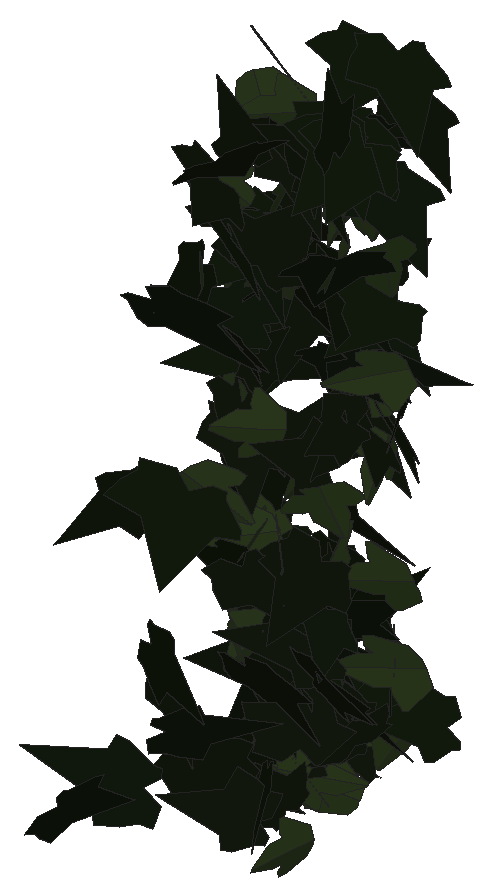
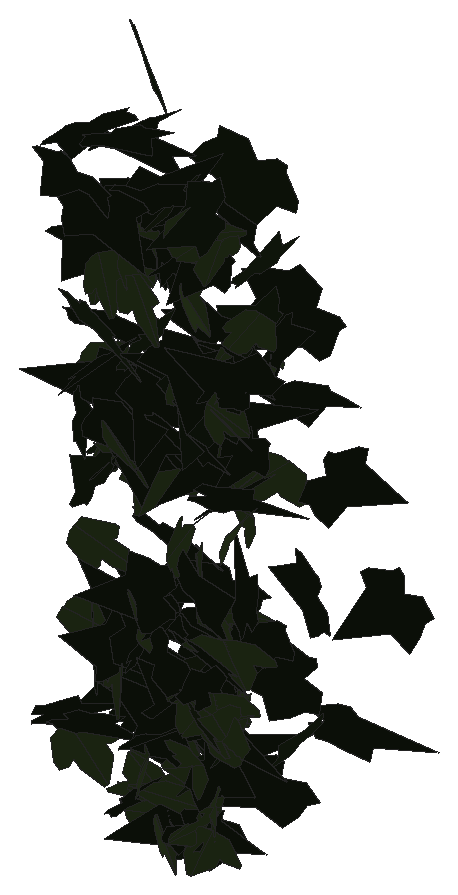
# SketchUp Ruby script. Lengths in inches.
U = 1.inch
M = Sketchup.active_model
def pt(a) = Geom::Point3d.new(a.map { |v| v * U })
def face(e, loops, mat)
  f = e.add_face(loops[0].map { |a| pt(a) })
  loops[1..].each { |l| e.add_face(l.map { |a| pt(a) }).erase! }
  f.material = f.back_material = mat if mat
  f
end
# faces: each face lists its corners as indices into pts; further lists are holes
def faces(e, pts, list, mat = nil) = list.each { |f| face(e, (f[0].is_a?(Array) ? f : [f]).map { |l| l.map { |i| pts[i] } }, mat) }
# xy, xz, yz: faces in a plane at the given z, y or x. An outline is a flat list of corners, or four numbers for a rectangle; further outlines are holes
def ring(l) = l.size == 4 ? [[l[0], l[1]], [l[2], l[1]], [l[2], l[3]], [l[0], l[3]]] : l.each_slice(2).to_a
def flat(e, list, mat, &to3) = list.each { |f| face(e, (f[0].is_a?(Array) ? f : [f]).map { |l| ring(l).map { |u, v| to3.(u, v) } }, mat) }
def xy(e, z, list, mat = nil) = flat(e, list, mat) { |x, y| [x, y, z] }
def xz(e, y, list, mat = nil) = flat(e, list, mat) { |x, z| [x, y, z] }
def yz(e, x, list, mat = nil) = flat(e, list, mat) { |y, z| [x, y, z] }
def lines(e, pts, list) = list.each { |a, b| e.add_line(pt(pts[a]), pt(pts[b])) }
# prism: a flat outline (further loops are holes) pulled along v
def prism(e, loops, v, mat = nil)
  f = face(e, loops, mat); d = Geom::Vector3d.new(v.map { |x| x * U })
  f.pushpull(f.normal.samedirection?(d) ? d.length : -d.length)
end
def box(e, o, s, mat = nil) = prism(e, [[o, [o[0] + s[0], o[1], o[2]], [o[0] + s[0], o[1] + s[1], o[2]], [o[0], o[1] + s[1], o[2]]]], [0, 0, s[2]], mat)
def at(x, y, z, deg = 0) = Geom::Transformation.translation(pt([x, y, z])) * Geom::Transformation.rotation(ORIGIN, Z_AXIS, deg.degrees)
def axes(o, x, y, z) = Geom::Transformation.new([*x, 0, *y, 0, *z, 0, *pt(o).to_a, 1])
def part(name) = M.definitions.add(name)
# library, detail: a bought-in or finely detailed component or shape, given as its bounding box
def library(name, o, s) = part(name).tap { |d| box(d.entities, o, s) }
def detail(e, o, s) = box(e.add_group.entities, o, s)
def put(e, d, t, mat = nil) = e.add_instance(d, t).tap { |i| i.material = mat if mat }
def group(e, t, mat = nil) = e.add_group.tap { |g| g.transformation = t; g.material = mat if mat }.entities
root = M.entities
M.materials.add("1026 AP 7946 SUNNY SIDE UP").color = [254, 231, 186]
M.materials.add("efeu1").color = [18, 25, 13]
M.materials.add("efeu2").color = [43, 57, 29]
c1 = part("ivyleaf_9")
p = [[1.54,2.16,1.25],[1.36,2.04,1.19],[-0.21,0.99,0.68],[-0.71,1.11,0.82],[-0.85,0.86,0.67],[-0.8,0.17,0.21],
  [-0.9,-0.01,0.1],[-0.67,-0.16,-0.02],[-0.08,-0.08,-0.05],[-0.03,-0.6,-0.4],[0.65,-0.88,-0.66],[0.83,-0.6,-0.49],
  [1.29,-0.42,-0.43],[1.8125,-0.07,-0.26],[1.21,0.44,0.15]]
faces(c1.entities,p,[[0,1,2,3,4,5,6,7,8,9,10,11,12,13,14]],"efeu1")
c2 = part("ivyleaf_10")
p = [[0,0.5,-0.03],[-0.0625,2.02,-0.43],[-0.19,2.01,-0.46],[-0.54,1.05,-0.29],[-0.52,0.625,-0.18],[-0.83,0.76,-0.28],
  [-1.16,0.64,-0.33],[-1.15,0.33,-0.24],[-0.77,-0.39,0.02],[-0.3,-0.51,0.16],[0.04,-0.48,0.23],[-0.02,2.01,-0.4375],
  [-0.06,2.01,-0.43],[0.04,-0.49,0.23],[0.67,-0.49,0.14],[1.38,0.36,-0.2],[1.375,0.51,-0.24],[0.81,0.65,-0.19],
  [0.62,0.59,-0.15],[0.6,1.09,-0.28],[0.5,1.23,-0.31]]
faces(c2.entities,p,[[0,1,2,3,4,5,6,7,8,9,10],[11,12,0,13,14,15,16,17,18,19,20]],"efeu2")
put(root,c1,axes([137.74,211.1,285.49],[-0.46349,-0.03246,0.23441],[-0.33897,-0.09016,-0.30122],[0.12619,-0.36141,0.05183]),"1026 AP 7946 SUNNY SIDE UP")
put(root,c2,axes([137.5625,210.79,284.78],[-0.00796,0.33057,-0.23303],[-0.14205,0.22131,0.33381],[0.61532,0.05537,0.07405]),"1026 AP 7946 SUNNY SIDE UP")
put(root,c1,axes([137.1875,210.96,283.58],[-0.03472,0.01197,0.4574],[0.05164,-0.44321,0.0114],[0.69637,0.03346,0.02196]),"1026 AP 7946 SUNNY SIDE UP")
put(root,c2,axes([137.37,211.12,283.06],[0.60482,0.09796,-0.04757],[-0.05306,-0.05562,-0.40657],[-0.1622,0.38346,-0.04438]),"1026 AP 7946 SUNNY SIDE UP")
put(root,c1,axes([137.98,208,280.22],[-0.34427,-0.14792,-0.33556],[-0.41907,-0.18582,0.2711],[-0.37342,0.3449,0.00512]),"1026 AP 7946 SUNNY SIDE UP")
put(root,c2,axes([137.5,211.23,287.08],[-0.01346,-0.25376,0.25977],[0.0236,-0.25371,-0.26249],[0.56362,0.00456,0.01719]),"1026 AP 7946 SUNNY SIDE UP")
put(root,c2,axes([137.33,210.61,288.33],[-0.17262,-0.24856,-0.23455],[0.26251,0.16626,-0.27064],[0.45871,-0.18869,0.06662]),"1026 AP 7946 SUNNY SIDE UP")
put(root,c1,axes([137.17,210.98,287.41],[-0.08394,0.02556,0.38678],[0.58508,0.05924,0.05072],[-0.08684,0.37442,-0.03217]),"1026 AP 7946 SUNNY SIDE UP")
put(root,c1,axes([137.31,209.54,280.79],[0.11048,-0.33291,0.09369],[0.01592,-0.09271,-0.35094],[0.54321,0.07043,-0.00877]),"1026 AP 7946 SUNNY SIDE UP")
put(root,c1,axes([137.71,208.33,284.62],[-0.11173,0.01078,-0.43675],[0.14962,-0.41855,-0.02984],[-0.64992,-0.09821,0.06821]),"1026 AP 7946 SUNNY SIDE UP")
put(root,c2,axes([137.57,211.21,281.84],[0.26628,0.25014,-0.15649],[-0.10126,-0.14103,-0.31112],[-0.45008,0.17972,-0.02259]),"1026 AP 7946 SUNNY SIDE UP")
put(root,c1,axes([138,210.9375,286.89],[-0.51521,0.09643,-0.21913],[-0.30085,0.10094,0.35046],[0.21195,0.37768,-0.03521]),"1026 AP 7946 SUNNY SIDE UP")
put(root,c2,axes([137.84,210.37,281.32],[-0.26236,0.30006,-0.21856],[-0.13006,0.19827,0.35423],[0.5646,0.1851,-0.01996]),"1026 AP 7946 SUNNY SIDE UP")
put(root,c1,axes([137.79,211.36,282.19],[0.00629,0.06183,0.33107],[-0.3689,-0.22304,0.04596],[0.35799,-0.23092,0.04155]),"1026 AP 7946 SUNNY SIDE UP")
put(root,c1,axes([138.09,210.49,286.42],[-0.18557,0.01426,0.38117],[-0.57425,-0.068,-0.11773],[0.09522,-0.38228,0.03285]),"1026 AP 7946 SUNNY SIDE UP")
put(root,c1,axes([137.62,210.12,282.93],[0.4821,0.12099,-0.13652],[-0.17707,-0.07626,-0.33883],[-0.2207,0.32547,-0.02637]),"1026 AP 7946 SUNNY SIDE UP")
put(root,c2,axes([137.47,210.6,285.07],[-0.18929,0.09258,-0.32433],[0.22353,-0.28813,-0.14474],[-0.46595,-0.17584,0.06232]),"1026 AP 7946 SUNNY SIDE UP")
put(root,c2,axes([137.86,211.07,281.86],[-0.39768,-0.24134,0.12812],[-0.11078,-0.10773,-0.35965],[0.41332,-0.26109,0.02688]),"1026 AP 7946 SUNNY SIDE UP")
put(root,c1,axes([137.63,209.79,287.46],[0.00424,-0.13917,-0.37407],[0.33016,-0.3042,0.1202],[-0.51327,-0.19682,0.07423]),"1026 AP 7946 SUNNY SIDE UP")
put(root,c2,axes([137.91,210.87,280],[-0.05666,0.08282,-0.37031],[-0.16778,0.34388,0.09453],[0.55598,0.11222,-0.00921]),"1026 AP 7946 SUNNY SIDE UP")
put(root,c1,axes([137.61,210.34,286.16],[0.50574,-0.0435,-0.13904],[-0.21337,0.00059,-0.33394],[0.06345,0.34871,-0.01471]),"1026 AP 7946 SUNNY SIDE UP")
put(root,c2,axes([137.64,211.06,289.73],[0.18859,0.35281,0.01986],[0.01968,0.01398,-0.38373],[-0.55507,0.12037,-0.00686]),"1026 AP 7946 SUNNY SIDE UP")
put(root,c1,axes([138.07,211.02,283.59],[0.04291,-0.00334,0.42526],[-0.24974,0.38178,0.01623],[-0.59916,-0.15937,0.02369]),"1026 AP 7946 SUNNY SIDE UP")
put(root,c2,axes([137.67,211.05,282.04],[0.54775,0.17392,-0.01781],[-0.00199,-0.03822,-0.39984],[-0.27498,0.34673,-0.03258]),"1026 AP 7946 SUNNY SIDE UP")
put(root,c2,axes([137.9,209.42,287.41],[0.04226,-0.17147,-0.32584],[-0.07619,0.31157,-0.17698],[0.55921,0.05541,0.00051]),"1026 AP 7946 SUNNY SIDE UP")
put(root,c2,axes([137.43,210.99,281.28],[-0.20885,0.03231,0.32991],[0.50582,0.01529,0.13602],[-0.00285,0.34619,-0.03476]),"1026 AP 7946 SUNNY SIDE UP")
put(root,c2,axes([137.77,211.15,279.69],[-0.47179,-0.05614,-0.07473],[0.12212,-0.02547,-0.31213],[0.076,-0.30756,0.03762]),"1026 AP 7946 SUNNY SIDE UP")
put(root,c1,axes([138.03,211.19,282.91],[-0.54347,0.02864,-0.07825],[0.11337,-0.04587,-0.35531],[-0.05918,-0.35093,0.03796]),"1026 AP 7946 SUNNY SIDE UP")
put(root,c1,axes([137.87,211.36,281.94],[-0.36309,0.0419,-0.23239],[0.30878,-0.13005,-0.23248],[-0.18728,-0.29564,0.06723]),"1026 AP 7946 SUNNY SIDE UP")
put(root,c2,axes([138.13,210.52,283.14],[-0.19304,0.03837,0.32138],[-0.25404,-0.29475,-0.0299],[0.42353,-0.1593,0.12855]),"1026 AP 7946 SUNNY SIDE UP")
put(root,c1,axes([138.11,210.84,287.74],[-0.6507,-0.11066,0.00159],[0.00984,-0.0318,-0.44023],[0.17376,-0.41261,0.0309]),"1026 AP 7946 SUNNY SIDE UP")
put(root,c1,axes([137.81,209.9375,288.78],[-0.16803,-0.25295,0.30816],[-0.00825,-0.31054,-0.27298],[0.61765,-0.07296,0.08019]),"1026 AP 7946 SUNNY SIDE UP")
put(root,c1,axes([137.56,210.3,287.93],[0.16366,-0.34602,0.26263],[0.15136,-0.23894,-0.37312],[0.66051,0.14049,0.02043]),"1026 AP 7946 SUNNY SIDE UP")
put(root,c2,axes([138.01,210.58,283.14],[0.15388,-0.36609,-0.06355],[-0.04168,0.05459,-0.38989],[0.58173,0.10075,-0.01113]),"1026 AP 7946 SUNNY SIDE UP")
put(root,c1,axes([137.94,210.94,280.86],[-0.13543,0.10288,-0.42709],[0.34317,-0.35365,-0.139],[-0.57841,-0.23391,0.01753]),"1026 AP 7946 SUNNY SIDE UP")
put(root,c1,axes([138.2,211.0625,279.73],[-0.10653,-0.00302,-0.32575],[-0.11717,-0.31411,0.01771],[-0.4832,0.07683,0.06753]),"1026 AP 7946 SUNNY SIDE UP")
put(root,c1,axes([137.95,211.05,287.76],[0.42562,0.25309,-0.12633],[-0.11842,-0.10082,-0.38173],[-0.42709,0.28017,-0.02006]),"1026 AP 7946 SUNNY SIDE UP")
put(root,c2,axes([137.85,210.93,279.84],[0.01901,-0.06443,-0.35492],[0.23727,0.31169,-0.05283],[0.49679,-0.1464,0.03882]),"1026 AP 7946 SUNNY SIDE UP")
put(root,c1,axes([137.66,211.17,290.33],[0.54574,-0.24878,-0.01932],[-0.05294,-0.0173,-0.43865],[0.38854,0.34708,-0.03263]),"1026 AP 7946 SUNNY SIDE UP")
put(root,c1,axes([138.48,210.42,281.23],[-0.08506,-0.04199,-0.40993],[-0.57758,-0.15339,0.06727],[-0.24852,0.37087,-0.01602]),"1026 AP 7946 SUNNY SIDE UP")
put(root,c2,axes([138.0625,210.62,281.58],[-0.09645,-0.19244,0.31027],[0.01895,-0.3076,-0.20103],[0.56313,-0.02261,0.0599]),"1026 AP 7946 SUNNY SIDE UP")
put(root,c1,axes([138.08,210.75,286.9],[0.14822,0.3837,0.18189],[0.08509,0.16619,-0.40588],[-0.65722,0.10805,-0.01153]),"1026 AP 7946 SUNNY SIDE UP")
put(root,c1,axes([137.78,210.375,285.3],[0.22904,-0.3355,-0.12077],[-0.05452,0.11061,-0.37596],[0.55516,0.14928,0.0129]),"1026 AP 7946 SUNNY SIDE UP")
put(root,c1,axes([138.3125,209.92,289.4],[0.09608,0.05621,0.36297],[-0.23109,0.32935,-0.02597],[-0.51066,-0.13847,0.08004]),"1026 AP 7946 SUNNY SIDE UP")
put(root,c1,axes([138.01,210.67,285.83],[0.07852,-0.02055,-0.36096],[-0.15318,0.33907,-0.03282],[0.53002,0.10104,0.04399]),"1026 AP 7946 SUNNY SIDE UP")
put(root,c1,axes([137.65,210.99,287.45],[0.27573,0.08668,-0.33673],[0.37047,0.23356,0.19509],[0.38246,-0.28872,0.05378]),"1026 AP 7946 SUNNY SIDE UP")
put(root,c1,axes([137.95,210.78,289.38],[0.53423,-0.05838,-0.08906],[-0.14166,-0.01799,-0.35371],[0.08182,0.35003,-0.03092]),"1026 AP 7946 SUNNY SIDE UP")
put(root,c2,axes([137.92,211.3125,280.97],[-0.28853,0.08538,-0.2564],[0.28985,-0.17561,-0.20271],[-0.29625,-0.25498,0.05139]),"1026 AP 7946 SUNNY SIDE UP")
put(root,c2,axes([138.37,210.98,289.62],[0.00829,0.01832,0.40061],[-0.19114,-0.36927,0.01747],[0.58135,-0.12167,0.00003]),"1026 AP 7946 SUNNY SIDE UP")
put(root,c2,axes([138.23,210.9375,287.19],[-0.19891,-0.36412,-0.07047],[0.04199,0.06095,-0.39672],[0.58045,-0.12919,0.00455]),"1026 AP 7946 SUNNY SIDE UP")
put(root,c1,axes([137.81,209.45,279.97],[0.05638,-0.02642,-0.44343],[0.26148,0.3992,-0.00864],[0.62538,-0.16453,0.04359]),"1026 AP 7946 SUNNY SIDE UP")
put(root,c1,axes([137.98,210.57,287.5625],[0.13358,-0.35145,0.02725],[-0.00048,-0.02933,-0.37259],[0.55443,0.08465,-0.00689]),"1026 AP 7946 SUNNY SIDE UP")
put(root,c1,axes([138.23,211.26,286.46],[-0.48512,-0.08538,-0.22038],[0.34945,-0.01945,-0.32305],[0.09241,-0.37465,0.06469]),"1026 AP 7946 SUNNY SIDE UP")
put(root,c1,axes([137.88,208.56,287.51],[0.69955,0.07432,0.10059],[0.162,-0.02968,-0.46251],[-0.10383,0.45442,-0.04392]),"1026 AP 7946 SUNNY SIDE UP")
put(root,c2,axes([138.3,210.92,288.6],[0.15943,-0.31654,0.12841],[0.03367,-0.12575,-0.34272],[0.53492,0.10226,-0.0167]),"1026 AP 7946 SUNNY SIDE UP")
put(root,c1,axes([138.03,210.87,280.66],[0.12269,-0.3446,0.15747],[0.0399,-0.15294,-0.36479],[0.59268,0.08163,-0.00804]),"1026 AP 7946 SUNNY SIDE UP")
put(root,c1,axes([138.14,210.1,284.91],[-0.04201,-0.40238,0.06028],[-0.0018,-0.06085,-0.41579],[0.63989,-0.02659,0.00279]),"1026 AP 7946 SUNNY SIDE UP")
put(root,c1,axes([138.02,211.01,279.68],[0.27349,-0.247,0.17069],[0.12197,-0.14931,-0.31142],[0.45276,0.18942,-0.01921]),"1026 AP 7946 SUNNY SIDE UP")
put(root,c1,axes([138.01,210.78,279.81],[0.04963,0.06052,-0.43509],[0.24736,0.39237,0.07227],[0.62417,-0.16031,0.00596]),"1026 AP 7946 SUNNY SIDE UP")
put(root,c2,axes([138.12,210.86,280],[-0.09705,-0.06156,0.38371],[0.43429,0.25044,0.09118],[-0.40546,0.28298,0.00581]),"1026 AP 7946 SUNNY SIDE UP")
put(root,c1,axes([138.29,210.7,281.47],[-0.26941,-0.02034,0.37963],[0.57082,0.0646,0.17788],[-0.10554,0.40132,-0.00698]),"1026 AP 7946 SUNNY SIDE UP")
put(root,c2,axes([138.31,208.85,284.75],[-0.36463,-0.17551,-0.27318],[0.39901,0.09365,-0.29303],[0.29918,-0.33881,0.05786]),"1026 AP 7946 SUNNY SIDE UP")
put(root,c1,axes([138.34,210.21,287.59],[-0.38467,0.15873,0.32272],[0.41895,-0.16314,0.29942],[0.3578,0.36167,-0.00363]),"1026 AP 7946 SUNNY SIDE UP")
put(root,c2,axes([138.61,211.17,279.61],[0.10706,-0.32773,0.00456],[-0.00681,-0.00732,-0.34483],[0.51538,0.06798,-0.00551]),"1026 AP 7946 SUNNY SIDE UP")
put(root,c1,axes([138.52,205.625,281.125],[-0.09422,0.14745,-0.41655],[-0.16546,0.3917,0.16517],[0.65748,0.1197,-0.01813]),"1026 AP 7946 SUNNY SIDE UP")
put(root,c1,axes([138.13,208.15,282.375],[0.10144,-0.10996,-0.41829],[0.65593,-0.0314,0.07697],[-0.07758,-0.40931,0.10389]),"1026 AP 7946 SUNNY SIDE UP")
put(root,c1,axes([138.65,208.91,289.84],[0.25671,0.43507,0.10699],[0.03686,0.09945,-0.47796],[-0.70146,0.16444,0.01404]),"1026 AP 7946 SUNNY SIDE UP")
put(root,c1,axes([138.26,208.35,281.02],[0.19599,0.25139,-0.30089],[0.11421,0.28765,0.28728],[0.59681,-0.1376,0.04384]),"1026 AP 7946 SUNNY SIDE UP")
put(root,c1,axes([138.47,210.72,289.17],[0.04945,-0.37759,-0.09211],[-0.01641,0.0867,-0.38981],[0.60915,0.03299,-0.00302]),"1026 AP 7946 SUNNY SIDE UP")
put(root,c2,axes([138.54,210.98,279.58],[0.30755,-0.16365,0.19821],[0.22564,-0.1297,-0.26341],[0.3282,0.24252,-0.00465]),"1026 AP 7946 SUNNY SIDE UP")
put(root,c2,axes([138.61,210.85,284.1],[0.00815,0.04029,0.39135],[0.25243,-0.34472,0.03341],[0.54466,0.15916,-0.02134]),"1026 AP 7946 SUNNY SIDE UP")
put(root,c2,axes([138.88,209.71,285.39],[-0.01957,0.11291,0.37513],[-0.09835,-0.35935,0.11068],[0.59037,-0.05612,0.03087]),"1026 AP 7946 SUNNY SIDE UP")
put(root,c1,axes([138.68,211.08,281.1],[-0.20491,-0.35436,-0.05746],[0.05061,0.0454,-0.38842],[0.5613,-0.13346,0.01405]),"1026 AP 7946 SUNNY SIDE UP")
put(root,c1,axes([138.35,211.05,281.26],[0.50353,0.03211,-0.2416],[0.34482,0.10906,0.32425],[0.14086,-0.38176,0.06988]),"1026 AP 7946 SUNNY SIDE UP")
put(root,c2,axes([139.16,211.12,288.5],[-0.40844,0.14317,0.23688],[-0.36623,0.04242,-0.29908],[-0.21529,-0.34376,0.05936]),"1026 AP 7946 SUNNY SIDE UP")
put(root,c1,axes([139.23,208.99,279.7],[-0.18214,-0.01626,0.37054],[-0.51746,-0.14873,-0.11695],[0.23002,-0.34746,0.03031]),"1026 AP 7946 SUNNY SIDE UP")
put(root,c1,axes([138.58,209.6,283.12],[-0.05901,-0.1318,-0.34169],[0.33712,0.25738,-0.12914],[0.44728,-0.21138,0.05226]),"1026 AP 7946 SUNNY SIDE UP")
put(root,c1,axes([138.93,210.82,286.75],[0.53076,-0.034,-0.26208],[-0.39818,0.02242,-0.34936],[0.06393,0.42197,-0.00007]),"1026 AP 7946 SUNNY SIDE UP")
put(root,c1,axes([139.01,211.3,282.42],[-0.11865,-0.05065,0.34679],[-0.24603,-0.30138,-0.08454],[0.47587,-0.16844,0.04276]),"1026 AP 7946 SUNNY SIDE UP")
put(root,c2,axes([138.7,210.11,283.32],[-0.01036,0.05558,0.36623],[0.39402,-0.25401,0.04425],[0.40532,0.24834,-0.03366]),"1026 AP 7946 SUNNY SIDE UP")
put(root,c1,axes([138.73,210.39,281.79],[0.09108,-0.33774,0.17569],[0.05595,-0.16885,-0.35396],[0.59367,0.06773,0.0064]),"1026 AP 7946 SUNNY SIDE UP")
put(root,c2,axes([138.92,211.26,280.67],[-0.2792,0.31833,-0.13124],[0.05096,-0.12927,-0.37475],[-0.53779,-0.17751,0.03262]),"1026 AP 7946 SUNNY SIDE UP")
put(root,c2,axes([139.35,210.73,279.4],[0.09615,0.09084,0.3421],[-0.44286,-0.17986,0.10323],[0.30995,-0.28517,0.04136]),"1026 AP 7946 SUNNY SIDE UP")
put(root,c1,axes([138.55,211.2,282.625],[-0.02312,-0.05097,-0.44311],[0.63311,0.15624,-0.03236],[0.24979,-0.40071,0.04101]),"1026 AP 7946 SUNNY SIDE UP")
put(root,c2,axes([138.84,210.96,280.1],[0.47203,0.16145,-0.18032],[0.20946,0.12136,0.34956],[0.31164,-0.32611,0.03817]),"1026 AP 7946 SUNNY SIDE UP")
put(root,c2,axes([138.96,211.1,282.8],[0.30047,-0.31017,0.07934],[-0.03649,0.07808,0.37516],[-0.50187,-0.19138,0.02023]),"1026 AP 7946 SUNNY SIDE UP")
put(root,c1,axes([138.62,211.22,283.54],[0.49627,-0.12807,0.17797],[0.23457,-0.09238,-0.35038],[0.24482,0.3481,-0.02505]),"1026 AP 7946 SUNNY SIDE UP")
put(root,c1,axes([139.11,207.64,285.35],[-0.51297,-0.30437,-0.11372],[0.18048,0.03521,-0.45642],[0.47505,-0.34204,0.0506]),"1026 AP 7946 SUNNY SIDE UP")
put(root,c1,axes([139.2,211.3,279.91],[-0.2026,-0.21398,0.24257],[-0.17411,-0.20939,-0.25836],[0.47052,-0.16962,0.00884]),"1026 AP 7946 SUNNY SIDE UP")
put(root,c2,axes([138.72,210.53,279.61],[0.08127,-0.06544,-0.35757],[0.5542,-0.00685,0.05542],[-0.02601,-0.35048,0.06356]),"1026 AP 7946 SUNNY SIDE UP")
put(root,c1,axes([138.93,209.24,281.84],[0.67435,-0.01437,-0.05097],[-0.0794,-0.03826,-0.44039],[0.01548,0.43,-0.03835]),"1026 AP 7946 SUNNY SIDE UP")
put(root,c1,axes([139.36,210.87,286.08],[0.4372,0.16547,-0.24735],[-0.29622,-0.15298,-0.33296],[-0.35156,0.33468,-0.02705]),"1026 AP 7946 SUNNY SIDE UP")
put(root,c1,axes([139.79,209.87,282.15],[-0.45597,0.10456,0.26977],[-0.41598,0.02664,-0.31331],[-0.15088,-0.38941,0.04855]),"1026 AP 7946 SUNNY SIDE UP")
put(root,c1,axes([139.51,210.43,289.4375],[0.01085,0.0372,0.45125],[-0.5692,-0.24771,0.02611],[0.39162,-0.36107,0.02545]),"1026 AP 7946 SUNNY SIDE UP")
put(root,c1,axes([139.19,209.28,280.25],[-0.22179,0.0379,-0.33948],[0.45133,-0.16598,-0.14712],[-0.26207,-0.31793,0.03394]),"1026 AP 7946 SUNNY SIDE UP")
put(root,c1,axes([139.61,209.17,279.95],[-0.08431,0.22915,0.28518],[-0.1569,0.25802,-0.23958],[-0.5412,-0.1105,0.02503]),"1026 AP 7946 SUNNY SIDE UP")
put(root,c1,axes([139.22,209.97,284.97],[-0.39456,0.32521,0.16515],[0.18786,-0.10753,0.42162],[0.53692,0.27661,-0.02616]),"1026 AP 7946 SUNNY SIDE UP")
put(root,c2,axes([139.62,210.96,281.93],[-0.28752,0.21273,0.24915],[-0.28296,0.1615,-0.28701],[-0.41832,-0.25546,0.02289]),"1026 AP 7946 SUNNY SIDE UP")
put(root,c2,axes([139.23,211.13,285.44],[0.5052,-0.19909,-0.0787],[0.14235,0.00449,0.38592],[-0.30289,-0.32996,0.0501]),"1026 AP 7946 SUNNY SIDE UP")
put(root,c1,axes([139.65,209.95,284.97],[-0.08654,-0.00456,0.36405],[-0.43184,-0.22458,-0.04836],[0.34981,-0.27837,0.03036]),"1026 AP 7946 SUNNY SIDE UP")
put(root,c1,axes([139.17,210.1875,289.58],[0.24612,-0.37953,0.04675],[0.00843,-0.04918,-0.42298],[0.60137,0.15602,-0.01321]),"1026 AP 7946 SUNNY SIDE UP")
put(root,c1,axes([139.31,210.76,287.29],[-0.02712,-0.30895,0.31104],[0.0054,-0.304,-0.3202],[0.68115,-0.00989,0.01492]),"1026 AP 7946 SUNNY SIDE UP")
put(root,c2,axes([139.5,210.79,288.84],[0.00012,-0.31615,0.23223],[0.0927,-0.22459,-0.32326],[0.60513,0.03447,0.04947]),"1026 AP 7946 SUNNY SIDE UP")
put(root,c1,axes([139.37,210.72,289.9],[-0.19872,-0.36804,-0.17816],[0.09616,0.15962,-0.39991],[0.63074,-0.14029,0.00484]),"1026 AP 7946 SUNNY SIDE UP")
put(root,c1,axes([139.6,209.5,280.79],[-0.42567,-0.14129,0.32846],[0.43176,0.16411,0.31528],[-0.33992,0.38539,-0.01086]),"1026 AP 7946 SUNNY SIDE UP")
put(root,c1,axes([139.64,211.03,290.92],[-0.37086,-0.28552,0.04915],[-0.02091,-0.05288,-0.38108],[0.45512,-0.23509,0.02254]),"1026 AP 7946 SUNNY SIDE UP")
put(root,c1,axes([139.79,211.18,289.79],[0.07326,0.25307,-0.26375],[-0.11732,-0.24724,-0.26572],[-0.5554,0.08561,0.02134]),"1026 AP 7946 SUNNY SIDE UP")
put(root,c1,axes([139.8,209.66,283.6],[-0.6379,-0.0347,-0.16893],[0.26114,-0.02914,-0.4176],[0.03327,-0.43653,0.03872]),"1026 AP 7946 SUNNY SIDE UP")
put(root,c1,axes([139.86,210.43,280.69],[-0.09164,-0.0289,0.36582],[-0.39274,-0.2535,-0.06494],[0.39984,-0.25563,0.02005]),"1026 AP 7946 SUNNY SIDE UP")
put(root,c2,axes([139.76,211.12,288.68],[-0.12353,-0.35787,0.00144],[0.01114,-0.00506,-0.37739],[0.56263,-0.07847,0.00779]),"1026 AP 7946 SUNNY SIDE UP")
put(root,c1,axes([139.36,210.4,282.27],[0.54715,0.19339,-0.08471],[0.08637,0.07201,0.40891],[0.31965,-0.35049,0.03451]),"1026 AP 7946 SUNNY SIDE UP")
put(root,c1,axes([139.61,210.85,282.14],[0.02047,0.03421,0.40083],[0.42434,0.28037,-0.03307],[-0.44356,0.2698,-0.01314]),"1026 AP 7946 SUNNY SIDE UP")
put(root,c1,axes([140.17,211.0625,287.8],[-0.30343,0.30702,0.11392],[-0.13814,0.07276,-0.37149],[-0.49321,-0.20926,0.03397]),"1026 AP 7946 SUNNY SIDE UP")
put(root,c1,axes([140.15,209.99,285.77],[-0.52646,0.19515,-0.01759],[-0.00292,-0.03915,-0.39786],[-0.30817,-0.33301,0.03382]),"1026 AP 7946 SUNNY SIDE UP")
put(root,c2,axes([139.79,209.78,284.63],[-0.36441,-0.2494,-0.11768],[0.16287,0.05693,-0.34852],[0.39841,-0.25139,0.03483]),"1026 AP 7946 SUNNY SIDE UP")
put(root,c1,axes([140.09,211.41,281.01],[-0.44518,-0.12955,0.157],[-0.20034,-0.08845,-0.32027],[0.24361,-0.30949,0.02354]),"1026 AP 7946 SUNNY SIDE UP")
put(root,c1,axes([139.65,210.79,285.37],[0.20499,-0.30725,-0.19246],[-0.09903,0.17425,-0.3427],[0.55524,0.14452,0.00993]),"1026 AP 7946 SUNNY SIDE UP")
put(root,c1,axes([139.47,210.13,281.42],[0.63622,-0.11581,0.05596],[0.07958,-0.02291,-0.43362],[0.18519,0.40769,-0.00589]),"1026 AP 7946 SUNNY SIDE UP")
put(root,c1,axes([139.74,209.91,282.72],[-0.07316,-0.33266,0.13812],[-0.01356,-0.13602,-0.3467],[0.56492,-0.04635,0.00957]),"1026 AP 7946 SUNNY SIDE UP")
put(root,c1,axes([140.28,209.83,280.89],[-0.08817,0.38184,0.17813],[-0.17948,0.15176,-0.38737],[-0.63274,-0.09626,0.08506]),"1026 AP 7946 SUNNY SIDE UP")
put(root,c2,axes([140.07,208.88,279.65],[0.01945,-0.05831,0.38278],[0.02192,-0.37177,-0.0627],[0.59151,0.01569,-0.01027]),"1026 AP 7946 SUNNY SIDE UP")
put(root,c2,axes([140.19,211.18,280.61],[-0.27676,-0.31879,0.1721],[-0.0805,-0.16391,-0.37473],[0.56151,-0.18063,0.0311]),"1026 AP 7946 SUNNY SIDE UP")
put(root,c1,axes([139.76,211.33,285.1],[0.13096,-0.25813,0.25278],[0.09193,-0.24019,-0.28048],[0.55402,0.10087,-0.01321]),"1026 AP 7946 SUNNY SIDE UP")
put(root,c1,axes([139.85,210.92,289.08],[-0.22546,-0.25998,-0.31754],[0.25772,0.2596,-0.30407],[0.57736,-0.21741,0.01173]),"1026 AP 7946 SUNNY SIDE UP")
put(root,c1,axes([139.87,210.92,287.04],[0.18142,-0.33185,-0.15801],[-0.04092,0.151,-0.36029],[0.57215,0.11603,0.02433]),"1026 AP 7946 SUNNY SIDE UP")
put(root,c1,axes([140.29,209.99,290.19],[-0.62368,-0.17665,-0.00552],[0.02464,-0.0245,-0.44647],[0.27675,-0.39591,0.0273]),"1026 AP 7946 SUNNY SIDE UP")
put(root,c1,axes([140.31,210.66,287.45],[-0.56537,-0.11549,0.00919],[0.0023,-0.03573,-0.38764],[0.18221,-0.3579,0.03341]),"1026 AP 7946 SUNNY SIDE UP")
put(root,c2,axes([140.23,209.6,288.58],[0.12815,-0.378,-0.09559],[-0.04772,0.08614,-0.39769],[0.60935,0.08624,-0.01104]),"1026 AP 7946 SUNNY SIDE UP")
put(root,c1,axes([139.7,210.54,286.38],[0.26847,0.11676,-0.35614],[0.30225,0.29647,0.20231],[0.48884,-0.24743,0.0705]),"1026 AP 7946 SUNNY SIDE UP")
put(root,c2,axes([140.47,210.43,286.5],[0.1644,0.0773,-0.35775],[-0.46293,-0.18521,-0.1347],[-0.31524,0.31229,0.01125]),"1026 AP 7946 SUNNY SIDE UP")
put(root,c1,axes([140.03,211.12,291],[-0.08123,-0.41957,-0.09459],[0.01571,0.08888,-0.43498],[0.67437,-0.05261,-0.00126]),"1026 AP 7946 SUNNY SIDE UP")
put(root,c2,axes([140.17,210.58,285.15],[-0.10535,-0.25894,0.27099],[0.20425,-0.26816,-0.23811],[0.54502,0.05044,0.14161]),"1026 AP 7946 SUNNY SIDE UP")
put(root,c1,axes([140.1,210.49,285.41],[-0.01623,-0.27319,0.21303],[0.03413,-0.20854,-0.28181],[0.53914,0.00498,0.02425]),"1026 AP 7946 SUNNY SIDE UP")
put(root,c2,axes([140.72,210.27,283.4],[-0.22359,0.00042,0.34573],[-0.50352,-0.10922,-0.14028],[0.15788,-0.34773,0.04224]),"1026 AP 7946 SUNNY SIDE UP")
put(root,c1,axes([140.48,209.23,288.77],[0.17451,0.37825,-0.1696],[-0.08198,-0.1585,-0.407],[-0.64482,0.12252,0.00584]),"1026 AP 7946 SUNNY SIDE UP")
put(root,c1,axes([140.18,210.77,281.4375],[0.01264,0.10933,0.40331],[-0.07312,-0.38812,0.11055],[0.63398,-0.04694,0.00471]),"1026 AP 7946 SUNNY SIDE UP")
put(root,c2,axes([140.39,210.3,288.4],[-0.2632,-0.3484,-0.11156],[0.09943,0.08743,-0.39723],[0.56406,-0.17798,0.01797]),"1026 AP 7946 SUNNY SIDE UP")
put(root,c1,axes([140.27,211.08,286],[-0.14495,-0.00674,-0.36037],[0.42794,-0.22865,-0.07069],[-0.34563,-0.28028,0.0636]),"1026 AP 7946 SUNNY SIDE UP")
put(root,c1,axes([140.375,209.9,290.2],[-0.25577,-0.3632,0.17456],[-0.05419,-0.17173,-0.40934],[0.62923,-0.16242,0.0357]),"1026 AP 7946 SUNNY SIDE UP")
put(root,c1,axes([140.14,211.29,290.21],[-0.24466,-0.09896,-0.34187],[0.50232,0.09779,-0.1841],[0.20792,-0.3527,0.04249]),"1026 AP 7946 SUNNY SIDE UP")
put(root,c2,axes([140.8125,210.29,282.06],[0.255,-0.0188,-0.36859],[-0.56294,0.0032,-0.16738],[0.01679,0.39271,-0.01398]),"1026 AP 7946 SUNNY SIDE UP")
put(root,c1,axes([140.05,209.29,282.04],[0.16915,-0.1642,0.31114],[0.27092,-0.24922,-0.20364],[0.46924,0.20308,0.00542]),"1026 AP 7946 SUNNY SIDE UP")
put(root,c1,axes([140.68,208.89,290.78],[0.00333,0.12779,0.44002],[-0.0444,0.42558,-0.12876],[-0.69852,-0.02644,0.01028]),"1026 AP 7946 SUNNY SIDE UP")
put(root,c1,axes([140.78,211.15,280.76],[-0.30078,-0.03748,0.29811],[-0.37176,-0.1833,-0.18639],[0.26947,-0.29471,0.0756]),"1026 AP 7946 SUNNY SIDE UP")
